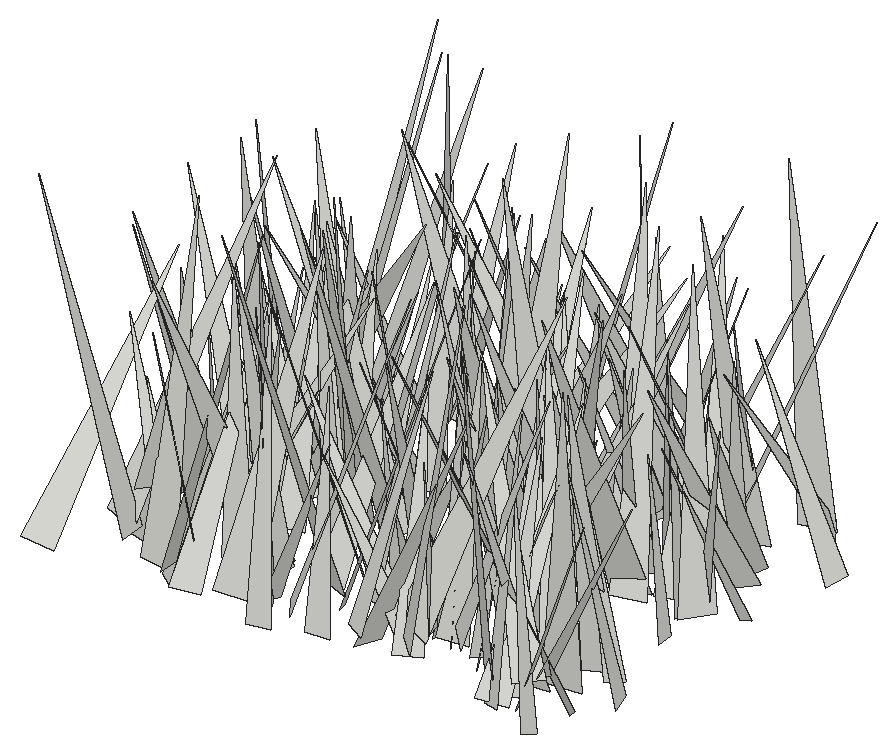
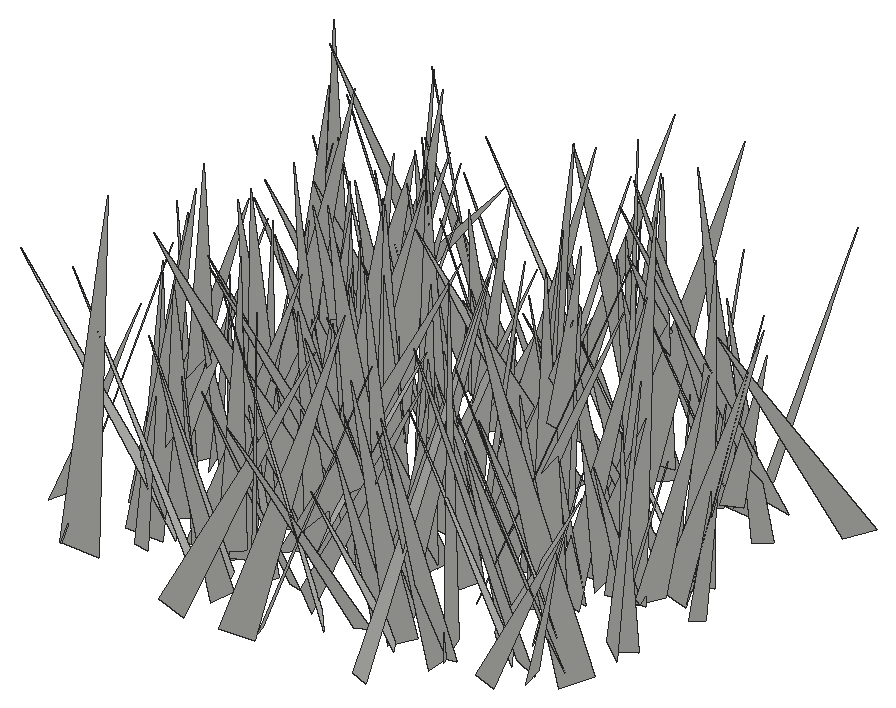
# SketchUp Ruby script. Lengths in inches.
U = 1.inch
M = Sketchup.active_model
def pt(a) = Geom::Point3d.new(a.map { |v| v * U })
def face(e, loops, mat)
  f = e.add_face(loops[0].map { |a| pt(a) })
  loops[1..].each { |l| e.add_face(l.map { |a| pt(a) }).erase! }
  f.material = f.back_material = mat if mat
  f
end
# faces: each face lists its corners as indices into pts; further lists are holes
def faces(e, pts, list, mat = nil) = list.each { |f| face(e, (f[0].is_a?(Array) ? f : [f]).map { |l| l.map { |i| pts[i] } }, mat) }
# xy, xz, yz: faces in a plane at the given z, y or x. An outline is a flat list of corners, or four numbers for a rectangle; further outlines are holes
def ring(l) = l.size == 4 ? [[l[0], l[1]], [l[2], l[1]], [l[2], l[3]], [l[0], l[3]]] : l.each_slice(2).to_a
def flat(e, list, mat, &to3) = list.each { |f| face(e, (f[0].is_a?(Array) ? f : [f]).map { |l| ring(l).map { |u, v| to3.(u, v) } }, mat) }
def xy(e, z, list, mat = nil) = flat(e, list, mat) { |x, y| [x, y, z] }
def xz(e, y, list, mat = nil) = flat(e, list, mat) { |x, z| [x, y, z] }
def yz(e, x, list, mat = nil) = flat(e, list, mat) { |y, z| [x, y, z] }
def lines(e, pts, list) = list.each { |a, b| e.add_line(pt(pts[a]), pt(pts[b])) }
# prism: a flat outline (further loops are holes) pulled along v
def prism(e, loops, v, mat = nil)
  f = face(e, loops, mat); d = Geom::Vector3d.new(v.map { |x| x * U })
  f.pushpull(f.normal.samedirection?(d) ? d.length : -d.length)
end
def box(e, o, s, mat = nil) = prism(e, [[o, [o[0] + s[0], o[1], o[2]], [o[0] + s[0], o[1] + s[1], o[2]], [o[0], o[1] + s[1], o[2]]]], [0, 0, s[2]], mat)
def at(x, y, z, deg = 0) = Geom::Transformation.translation(pt([x, y, z])) * Geom::Transformation.rotation(ORIGIN, Z_AXIS, deg.degrees)
def axes(o, x, y, z) = Geom::Transformation.new([*x, 0, *y, 0, *z, 0, *pt(o).to_a, 1])
def part(name) = M.definitions.add(name)
# library, detail: a bought-in or finely detailed component or shape, given as its bounding box
def library(name, o, s) = part(name).tap { |d| box(d.entities, o, s) }
def detail(e, o, s) = box(e.add_group.entities, o, s)
def put(e, d, t, mat = nil) = e.add_instance(d, t).tap { |i| i.material = mat if mat }
def group(e, t, mat = nil) = e.add_group.tap { |g| g.transformation = t; g.material = mat if mat }.entities
root = M.entities
c1 = part("fur_instance\#9")
p = [[0.8125,0,1.79],[0.67,-0.02,1.48],[0,-0.11,0],[0,0.11,0]]
faces(c1.entities,p,[[0,1,2,3]])
put(root,c1,axes([119.71,154.68,-28.22],[3.07442,-7.15508,0.96712],[-6.88437,-3.22185,-1.95131],[-2.1762,0.08396,7.5392]))
put(root,c1,axes([124.55,151.32,-28.22],[-0.37436,4.96388,1.61425],[5.21969,0.34743,0.14211],[-0.02763,-1.62026,4.97594]))
put(root,c1,axes([133.8,152.13,-28.22],[4.65437,1.55789,0.49043],[1.62302,-4.57734,-0.86283],[-0.1826,-0.97553,4.83174]))
put(root,c1,axes([115.31,151.59,-27.1],[-7.20158,-1.52489,0.67202],[-1.60184,7.15641,-0.92717],[0.45935,1.04894,7.30263]))
put(root,c1,axes([117.04,153.1,-27.1],[-3.29784,-3.61715,1.25797],[-3.53735,3.51322,0.8285],[1.46745,0.33986,4.82422]))
put(root,c1,axes([132.45,151.96,-28.22],[3.92843,5.06138,3.38638],[5.5366,-4.64662,0.52215],[-2.53598,-2.30413,6.38572]))
put(root,c1,axes([119.68,149.32,-27.1],[-3.94963,4.34285,0.40783],[4.0226,3.83915,-1.92507],[1.68683,1.01332,5.54563]))
put(root,c1,axes([124.15,152.97,-27.1],[-4.11377,-6.51171,1.45116],[-6.65439,3.88319,-1.43913],[-0.47668,1.98739,7.56666]))
put(root,c1,axes([122.36,150.46,-28.22],[0.64289,6.12986,1.03372],[6.0316,-0.86662,1.38779],[-1.50455,-0.85491,6.00521]))
put(root,c1,axes([135.55,150.41,-28.22],[-4.92435,-0.05312,0.24709],[-0.15186,4.47527,-2.06445],[0.20202,2.06935,4.47102]))
put(root,c1,axes([121.42,152.375,-28.22],[4.16125,-1.09144,0.28201],[-1.11074,-4.15389,0.31328],[-0.19241,0.37504,4.29058]))
put(root,c1,axes([114.2,153.07,-28.22],[0.76926,-4.66703,1.07076],[-4.59745,-0.41678,1.48633],[1.33832,1.25083,4.49041]))
put(root,c1,axes([127.77,152.92,-28.22],[-4.18794,0.93567,0.33129],[0.9893,4.05153,1.06324],[0.08071,-1.11073,4.15738]))
put(root,c1,axes([126.38,152.1,-28.22],[6.16079,-1.33707,0.34037],[-1.37023,-6.11166,0.79308],[-0.16154,0.84778,6.25413]))
put(root,c1,axes([118.02,150.41,-27.1],[6.46332,2.41268,1.62775],[2.03661,-6.58136,1.66821],[-2.07914,1.05343,6.69422]))
put(root,c1,axes([128.95,151.23,-27.1],[4.76999,5.26227,1.90717],[5.37132,-5.00824,0.38463],[-1.57405,-1.14351,7.09199]))
put(root,c1,axes([126.68,150.94,-27.1],[2.68207,4.86571,0.6841],[4.89534,-2.71316,0.10499],[-0.42283,-0.54794,5.55496]))
put(root,c1,axes([119.82,152.41,-27.1],[-1.05184,5.80364,2.59591],[6.34975,1.09094,0.13387],[0.3189,-2.57972,5.89666]))
put(root,c1,axes([133.72,153.375,-28.22],[-1.08629,-5.09453,1.21583],[-5.17343,0.84989,-1.06105],[-0.81738,1.39139,5.09985]))
put(root,c1,axes([117.41,152.12,-28.22],[-3.05082,2.35934,0.28628],[2.37608,3.01778,0.45074],[-0.05159,-0.53147,3.83025]))
put(root,c1,axes([123.64,150.8,-27.1],[5.3948,4.35682,0.5893],[4.31887,-5.42625,0.57994],[-0.82254,0.08385,6.9101]))
put(root,c1,axes([116.4,151.8,-28.22],[0.76042,7.54721,2.45249],[7.93568,-0.724,-0.23253],[-0.00259,-2.46349,7.58186]))
put(root,c1,axes([121.46,152.47,-28.22],[4.32475,3.25099,2.86901],[3.37923,-5.06616,0.64681],[-2.71679,-1.12634,5.37159]))
put(root,c1,axes([117.27,151.1875,-28.22],[2.99735,3.72962,0.28981],[3.68324,-3.00724,0.60693],[-0.65404,0.15682,4.74613]))
put(root,c1,axes([134.3,153.97,-28.22],[2.16747,-6.96935,1.82134],[-7.20329,-2.08612,0.58967],[0.04123,1.91397,7.27476]))
put(root,c1,axes([128.99,152.79,-27.1],[3.01328,1.01562,1.71575],[1.06477,-3.44849,0.1713],[-1.68569,-0.36275,3.17522]))
put(root,c1,axes([133.1,151.16,-28.22],[2.56304,5.03632,1.18387],[4.82189,-2.80423,1.49027],[-1.87495,-0.32715,5.45094]))
put(root,c1,axes([120.19,151.72,-28.22],[-2.56408,6.91655,2.55207],[6.94878,3.17004,-1.60986],[2.46298,-1.74312,7.19872]))
put(root,c1,axes([130.14,152.91,-27.1],[4.42305,4.26534,0.99754],[4.37397,-4.22348,-1.33498],[0.23791,-1.64944,5.99786]))
put(root,c1,axes([135.9,152.64,-28.22],[-5.38862,-5.55187,0.24968],[-4.68183,4.34761,-4.37054],[-2.99434,3.19341,6.38427]))
put(root,c1,axes([120.52,154.02,-28.22],[-6.63003,0.58928,2.6026],[0.94805,7.03587,0.82207],[2.49439,-1.10786,6.6052]))
put(root,c1,axes([133.06,152.06,-28.22],[-4.05743,3.11883,1.27429],[2.94276,4.25195,-1.03673],[1.64046,0.08657,5.0115]))
put(root,c1,axes([111.75,150.27,-28.22],[-2.9172,5.75801,0.16061],[5.28877,2.74872,-2.48273],[2.2824,0.99014,5.95825]))
put(root,c1,axes([128.23,152.23,-28.22],[-2.91757,4.706,0.99504],[4.75363,2.9987,-0.24403],[0.73452,-0.71423,5.53165]))
put(root,c1,axes([134.27,152.02,-27.1],[-2.5947,5.83184,0.30944],[5.66182,2.42897,1.69778],[-1.43174,-0.96349,6.15308]))
put(root,c1,axes([130.73,153.38,-28.22],[3.30079,2.00098,0.99665],[2.11543,-3.37049,-0.23912],[-0.72261,-0.72685,3.85253]))
put(root,c1,axes([115.67,153.16,-27.1],[-2.80157,3.07223,0.58027],[3.12461,2.72376,0.66487],[-0.11008,-0.87559,4.10431]))
put(root,c1,axes([134.52,152.61,-27.1],[4.0884,0.15219,0.34801],[0.0557,-3.96154,1.07814],[-0.37573,1.0688,3.94662]))
put(root,c1,axes([128.25,152.37,-27.1],[1.6055,7.88479,1.47704],[7.72527,-1.11383,-2.45126],[2.16141,-1.87581,7.66412]))
put(root,c1,axes([123.74,155.37,-28.22],[-4.79453,-5.10071,1.01007],[-5.15614,4.84133,-0.02673],[0.67211,0.75447,7.00029]))
put(root,c1,axes([129.76,155.625,-28.22],[5.66121,2.03663,0.41958],[1.99596,-4.98096,-2.75306],[0.58316,-2.72311,5.34956]))
put(root,c1,axes([136.84,154.43,-28.22],[-4.98874,-1.77944,1.14235],[-1.81158,5.1064,0.04294],[1.09068,0.3424,5.29642]))
put(root,c1,axes([132.96,151.43,-28.22],[-3.49002,4.97532,0.38419],[4.70613,3.43753,-1.76559],[1.65943,0.71499,5.81522]))
put(root,c1,axes([118.51,155.99,-28.22],[-4.19902,-6.23031,2.61813],[-6.01537,4.8505,1.89504],[3.08005,0.97931,7.27031]))
put(root,c1,axes([128.82,154.14,-28.22],[-1.46748,5.77462,2.34569],[6.13429,1.76496,-0.50731],[1.10405,-2.13089,5.93652]))
put(root,c1,axes([128.125,154.48,-28.22],[5.41159,0.09186,1.28906],[0.07062,-5.56242,0.09991],[-1.29039,0.08081,5.41145]))
put(root,c1,axes([134.69,155.86,-28.22],[2.11565,-6.08651,1.80009],[-6.2822,-2.27872,-0.32139],[-0.90548,1.58863,6.43571]))
put(root,c1,axes([117.9,155.93,-28.22],[5.48101,-1.25937,0.85366],[-1.15676,-5.52263,-0.72019],[-0.98826,-0.52035,5.57753]))
put(root,c1,axes([114.3,152.17,-27.1],[2.50136,7.65725,0.1478],[7.63522,-2.48107,-0.67805],[0.59891,-0.35058,8.02686]))
put(root,c1,axes([117.74,154.5,-28.22],[3.45283,2.51437,0.03768],[2.48973,-3.40925,-0.65094],[0.3531,-0.54815,4.22141]))
put(root,c1,axes([124.81,155.34,-28.22],[-4.21656,2.08304,0.19454],[2.06998,4.09043,1.06765],[-0.30342,-1.04195,4.58024]))
put(root,c1,axes([129.93,157.18,-28.22],[-3.59271,-3.52154,0.36411],[-3.38524,3.56898,1.11534],[1.03633,-0.55007,4.90559]))
put(root,c1,axes([135.59,155.59,-28.22],[1.42768,-3.34431,1.65268],[-3.54003,-1.77266,-0.52903],[-1.17641,1.27565,3.59761]))
put(root,c1,axes([125.07,157.35,-28.22],[-0.67207,-6.04885,0.74296],[-6.03248,0.76649,0.78356],[0.86591,0.6451,6.03542]))
put(root,c1,axes([131,156.88,-28.22],[-0.74587,-6.40704,1.23448],[-6.45249,0.53969,-1.09751],[-0.96927,1.33753,6.35625]))
put(root,c1,axes([113.98,157.4,-28.22],[4.76035,-4.27512,0.72339],[-4.20428,-4.81383,-0.78223],[-1.06017,-0.10597,6.35025]))
put(root,c1,axes([128.85,154.05,-28.22],[5.31118,5.11176,2.74997],[4.78098,-5.96627,1.85658],[-3.29161,-0.41778,7.13385]))
put(root,c1,axes([130.91,155.34,-28.22],[-7.32876,-0.97242,0.83606],[-1.07916,7.29688,-0.97277],[0.69283,1.07947,7.32872]))
put(root,c1,axes([123.52,157.71,-28.22],[-2.25691,-7.5793,1.44794],[-7.71352,2.17504,-0.63772],[-0.20948,1.56823,7.88243]))
put(root,c1,axes([126.92,156.79,-28.22],[-3.55918,-3.90599,0.48478],[-3.91702,3.45103,-0.95229],[-0.38568,0.99656,5.19785]))
put(root,c1,axes([130.33,153.8,-28.22],[1.86893,4.92203,0.04113],[4.36091,-1.67616,2.42774],[-2.28266,0.8277,4.67176]))
put(root,c1,axes([126.48,157.73,-28.22],[4.05285,-0.43746,0.41546],[-0.3233,-3.95717,-1.01285],[-0.50937,-0.96903,3.94856]))
put(root,c1,axes([124.16,156.61,-28.22],[0.90627,3.33198,1.59944],[3.57947,-1.20149,0.47479],[-0.9207,-1.39138,3.42023]))
put(root,c1,axes([113.74,158.14,-28.22],[-5.14482,-3.13912,1.24988],[-3.04737,5.29445,0.7535],[1.4594,-0.01101,5.97959]))
put(root,c1,axes([115.6,156.49,-28.22],[-3.72029,-1.54775,1.40082],[-1.82397,3.80239,-0.64288],[1.01535,1.15959,3.97778]))
put(root,c1,axes([132.49,155.91,-28.22],[-2.14866,5.91991,1.32548],[6.06222,2.04254,0.70466],[-0.22751,-1.48381,6.25824]))
put(root,c1,axes([123.9,153.63,-28.22],[6.2923,4.31715,0.79405],[3.75537,-6.01297,2.93303],[-2.27277,2.01685,7.04472]))
put(root,c1,axes([119.83,159.88,-28.22],[-1.88375,-7.99896,1.23534],[-7.80751,2.13018,1.88761],[2.13359,0.73274,7.99805]))
put(root,c1,axes([126.28,157.98,-28.22],[4.01557,-5.25956,2.05629],[-5.53772,-4.16187,0.169],[-1.10676,1.74125,6.61508]))
put(root,c1,axes([124.33,154.78,-28.22],[3.92721,6.27569,0.86047],[6.07775,-4.01843,1.56873],[-1.78486,0.12492,7.23508]))
put(root,c1,axes([127.15,160.48,-28.22],[4.78768,-6.87101,0.53821],[-6.76798,-4.81092,-1.21319],[-1.30189,-0.25808,8.28619]))
put(root,c1,axes([114.15,158.61,-28.22],[-0.64276,-5.9949,1.38637],[-6.03632,0.34404,-1.31091],[-1.1932,1.48889,5.88502]))
put(root,c1,axes([122.42,154.625,-28.22],[-4.56425,4.1816,0.8559],[3.58274,4.43445,-2.55936],[2.31998,1.37862,5.63629]))
put(root,c1,axes([116.25,156.52,-28.22],[2.28513,5.39499,0.34939],[5.12885,-2.04337,-1.99232],[1.70965,-1.08097,5.50984]))
put(root,c1,axes([112.37,159.34,-28.22],[4.01864,-1.00258,0.99057],[-0.63294,-3.95809,-1.43832],[-1.25928,-1.21004,3.88405]))
put(root,c1,axes([121.36,157.57,-28.22],[-6.31517,-2.67121,2.41272],[-3.08957,6.52254,-0.86542],[1.84694,1.77736,6.80204]))
put(root,c1,axes([128.8125,158.05,-28.22],[4.74645,-3.63152,0.20608],[-3.44873,-4.38539,2.15263],[1.15614,1.82746,5.57521]))
put(root,c1,axes([121.21,156.54,-28.22],[-6.71,0.21588,0.88951],[-0.0468,6.49159,-1.92847],[0.91413,1.91692,6.43053]))
put(root,c1,axes([118.56,157.11,-28.22],[-1.85743,4.94831,0.92273],[4.99711,1.93095,-0.29602],[0.60509,-0.75691,5.27714]))
put(root,c1,axes([131.72,161.43,-28.22],[2.00321,-7.73932,0.37509],[-7.71802,-2.02729,-0.61059],[-0.68548,0.20889,7.97102]))
put(root,c1,axes([123.2,159.25,-28.22],[1.52564,-3.34819,0.07276],[-3.07421,-1.36842,1.48995],[1.32851,0.67846,3.36423]))
put(root,c1,axes([129.36,159.05,-28.22],[-2.05605,-4.2865,1.82271],[-4.5186,2.31917,0.35698],[1.13077,1.47345,4.74068]))
put(root,c1,axes([115.48,159.86,-28.22],[1.30407,-7.61557,2.3618],[-7.95747,-1.39423,-0.10194],[-0.50366,2.30972,7.72574]))
put(root,c1,axes([130.09,158.49,-28.22],[2.97809,2.23148,0.68885],[2.24903,-3.04112,0.12836],[-0.62921,-0.30835,3.71915]))
put(root,c1,axes([130.51,156.68,-28.22],[-3.78371,6.02543,0.57396],[5.96039,3.82698,-0.88298],[1.05307,-0.01122,7.05993]))
put(root,c1,axes([122.22,160.31,-28.22],[-3.95359,-4.39819,1.62013],[-4.4402,4.19331,0.54823],[1.50116,0.81969,5.8885]))
put(root,c1,axes([135.09,159.27,-28.22],[-3.75742,-0.36081,1.22113],[-0.40687,3.94545,-0.08619],[1.20657,0.20686,3.77372]))
put(root,c1,axes([128.77,161.64,-28.22],[1.34944,-6.66989,1.0863],[-6.57389,-1.5523,-1.36482],[-1.56569,0.76902,6.66676]))
put(root,c1,axes([128.64,158.72,-28.22],[-2.07994,4.49979,1.08625],[4.57933,2.1742,-0.23818],[0.67657,-0.88257,4.95151]))
put(root,c1,axes([128.86,162,-28.22],[3.45501,-4.88886,0.26504],[-4.85303,-3.46254,-0.60598],[-0.64754,-0.13474,5.95575]))
put(root,c1,axes([114.7,159.34,-28.22],[-5.78073,2.46703,0.60773],[2.49572,5.79658,0.20851],[0.47643,-0.43109,6.28168]))
put(root,c1,axes([122.02,159.32,-28.22],[-1.88222,6.06948,1.49765],[6.0067,1.32242,2.18977],[-1.73238,-2.00921,5.96542]))
put(root,c1,axes([117.15,161.375,-28.22],[-1.29627,-6.42722,1.30707],[-6.54569,1.18361,-0.67151],[-0.41416,1.4099,6.52216]))
put(root,c1,axes([116.67,161.05,-28.22],[3.94876,4.2171,2.00571],[4.64379,-3.26946,-2.26834],[0.4919,-2.98768,5.31331]))
put(root,c1,axes([119.9,163.24,-28.22],[-6.16351,-3.9605,0.27898],[-3.73191,5.95492,2.08903],[1.35509,-1.6142,7.02213]))
put(root,c1,axes([128.67,161.89,-28.22],[3.0521,-3.8403,0.46149],[-3.78154,-3.08617,-0.67208],[-0.8129,-0.06212,4.85917]))
put(root,c1,axes([117.58,159.29,-28.22],[-2.49681,4.68547,0.3153],[4.52882,2.308,1.56527],[-1.24213,-1.0033,5.07323]))
put(root,c1,axes([119.26,160.23,-28.22],[3.71191,-5.65782,4.04126],[-6.28277,-4.69165,-0.79764],[-2.97818,2.84578,6.7196]))
put(root,c1,axes([130.11,159.36,-28.22],[-3.95695,1.67084,0.9926],[1.45221,4.03835,-1.00857],[1.29152,0.5783,4.17516]))
put(root,c1,axes([120.74,160.68,-28.22],[-7.40149,0.22253,0.007],[0.22253,7.40149,0.00759],[0.00677,-0.0078,7.40483]))
put(root,c1,axes([117.37,162.16,-28.22],[5.14782,-4.26055,1.16689],[-4.27581,-5.25589,-0.32723],[-1.10966,0.4872,6.67423]))
put(root,c1,axes([127.77,162.71,-28.22],[7.05622,-1.23215,0.51957],[-1.10047,-6.93599,-1.50315],[-0.75967,-1.39725,7.0035]))
put(root,c1,axes([114.68,161.1875,-28.22],[-3.79015,-1.11399,0.60809],[-1.15598,3.82064,-0.20588],[0.52388,0.37109,3.9451]))
put(root,c1,axes([134.41,162.47,-28.22],[-1.98967,-4.65459,1.69235],[-4.24096,2.54317,2.00863],[2.55803,0.59592,4.64644]))
put(root,c1,axes([125.39,162.07,-28.22],[0.0585,-4.06465,0.78718],[-4.11626,0.02739,0.44734],[0.44434,0.78888,4.04038]))
put(root,c1,axes([130.58,162.91,-28.22],[-0.89521,-5.51634,1.09126],[-5.41102,1.14576,1.35291],[1.53027,0.82431,5.42227]))
put(root,c1,axes([114.91,160.12,-28.22],[-3.70619,1.07071,1.22273],[0.63141,3.75399,-1.37341],[1.4976,1.06701,3.605]))
put(root,c1,axes([127.24,162.42,-28.22],[3.59874,-6.83955,3.08177],[-7.12327,-4.18751,-0.97538],[-2.35281,2.21652,7.66674]))
put(root,c1,axes([125.36,161.66,-28.22],[-2.45983,6.23998,3.07468],[6.83629,2.77173,-0.15592],[1.28687,-2.79677,6.7055]))
put(root,c1,axes([112.89,162.89,-28.22],[0.91273,-4.1627,0.50654],[-4.12867,-0.80133,0.85424],[0.734,0.66898,4.1751]))
put(root,c1,axes([116.97,159.14,-28.22],[-5.60466,1.1961,0.32776],[0.92969,5.05609,-2.5538],[0.82084,2.4404,5.13039]))
put(root,c1,axes([124.52,162.26,-28.22],[7.01983,-0.71592,2.31882],[-0.6287,-7.39114,-0.37866],[-2.34397,-0.1616,7.04608]))
put(root,c1,axes([134.81,164.43,-28.22],[2.61621,-5.42084,0.25429],[-5.22177,-2.59146,-1.52055],[-1.47757,-0.43991,5.82391]))
put(root,c1,axes([136.47,162.45,-28.22],[-1.27388,-3.61865,0.59779],[-3.46584,0.98064,-1.44951],[-1.19998,1.0092,3.55195]))
put(root,c1,axes([124.6875,159.98,-28.22],[-0.78819,5.89997,0.04998],[5.7265,0.75282,1.4401],[-1.42105,-0.23877,5.77555]))
put(root,c1,axes([118.28,161.37,-28.22],[-1.7521,4.37342,1.24469],[4.49457,1.86786,-0.23622],[0.6891,-1.06311,4.7054]))
put(root,c1,axes([134.89,161.49,-28.22],[-6.12251,3.37612,2.03098],[3.42132,6.417,-0.35327],[1.95387,-0.65732,6.98272]))
put(root,c1,axes([123.3,162.42,-28.22],[-0.9402,5.50023,2.63792],[6.09336,0.97222,0.14463],[0.28664,-2.62629,5.57814]))
put(root,c1,axes([122.62,162.35,-28.22],[4.20762,-3.32651,0.12048],[-3.15177,-3.91891,1.86887],[1.07075,1.53645,5.02763]))
put(root,c1,axes([128.79,160.3125,-28.22],[2.4518,5.85296,0.01413],[5.81055,-2.43218,-0.76857],[0.70347,-0.30989,6.29903]))
put(root,c1,axes([131.66,163.125,-28.22],[-0.88602,-4.48963,1.06047],[-4.46813,0.56653,-1.33464],[-1.14769,1.26043,4.37728]))
put(root,c1,axes([117.72,161.5625,-28.22],[4.17653,-0.25853,0.87813],[-0.4857,-4.1025,1.10224],[-0.77592,1.17643,4.03674]))
put(root,c1,axes([134.42,161.11,-28.22],[-5.22043,-0.84385,1.05571],[-1.17009,4.93002,-1.84535],[0.67639,2.01552,4.95577]))
put(root,c1,axes([131.96,160.95,-28.22],[-1.2461,7.24945,1.28302],[7.36015,1.19663,0.38699],[-0.1701,-1.32928,7.34558]))
put(root,c1,axes([128.54,161.49,-28.22],[-3.66348,3.88372,0.60062],[3.90017,3.69385,-0.09601],[0.48235,-0.37054,5.33808]))
put(root,c1,axes([132.22,162.94,-28.22],[4.15283,1.56186,1.94961],[1.7605,-4.5132,-0.13443],[-1.7723,-0.82343,4.43479]))
put(root,c1,axes([134.49,165.39,-28.22],[4.609,-3.3139,0.05026],[-3.15306,-4.41083,-1.68231],[-1.0211,-1.33793,5.42168]))
put(root,c1,axes([133.01,161.88,-28.22],[-1.57636,3.66287,0.67143],[3.67727,1.64614,-0.34684],[0.58749,-0.47537,3.97256]))
put(root,c1,axes([125.1875,163.32,-28.22],[4.4628,-4.8312,0.78242],[-4.8199,-4.15484,1.83716],[0.84924,1.80724,6.31521]))
put(root,c1,axes([126.52,163.34,-28.22],[3.82808,-2.96393,0.87418],[-3.08142,-3.76593,0.72521],[-0.23226,1.11183,4.78677]))
put(root,c1,axes([128.93,163.4375,-28.22],[3.70956,-2.15387,1.10856],[-2.28011,-3.78925,0.26761],[-0.81802,0.79458,4.28116]))
put(root,c1,axes([123.57,163.13,-28.22],[-3.05036,2.77962,1.08054],[2.93347,3.07501,0.37088],[0.53722,-1.00823,4.11016]))
put(root,c1,axes([113.43,163.22,-28.22],[-3.6941,-4.73944,2.34113],[-5.23892,3.66336,-0.85037],[0.70493,2.38895,5.94858]))
put(root,c1,axes([133.71,165.77,-28.22],[-3.10911,-5.59083,0.18925],[-5.58666,3.11434,0.22319],[0.28707,0.05678,6.39328]))
put(root,c1,axes([127.66,164.66,-28.22],[-7.5943,2.08618,0.38061],[2.11361,7.33132,1.9887],[-0.17228,-2.01745,7.62041]))
put(root,c1,axes([116.26,164.46,-28.22],[-3.02688,-2.08558,0.64094],[-2.07151,3.09116,0.27563],[0.68504,0.13224,3.66547]))
put(root,c1,axes([112.98,165.95,-28.22],[2.01455,-7.63294,0.11302],[-6.59973,-1.68273,3.99311],[3.83642,1.11337,6.80994]))
put(root,c1,axes([122.57,165.05,-28.22],[-6.83352,3.26319,2.339],[3.80782,6.73136,1.73366],[1.27275,-2.61852,7.37155]))
put(root,c1,axes([130.33,162.99,-28.22],[-5.59489,5.13542,2.2708],[5.22691,5.9344,-0.54239],[2.05147,-1.11455,7.57503]))
put(root,c1,axes([118.36,162.66,-28.22],[5.33264,0.16428,1.51785],[-0.27785,-5.31816,1.55174],[-1.50122,1.56784,5.10452]))
put(root,c1,axes([120.87,162.73,-28.22],[-5.25856,3.05312,1.43062],[2.8843,5.44607,-1.02073],[1.74617,0.1987,5.99435]))
put(root,c1,axes([126.7,164.37,-28.22],[3.66382,-3.28739,1.57998],[-3.52995,-3.75957,0.36325],[-0.918,1.33625,4.90903]))
put(root,c1,axes([128.91,166.47,-28.22],[4.74802,-2.11154,0.82126],[-1.70244,-4.58339,-1.94189],[-1.49491,-1.48682,4.81989]))
put(root,c1,axes([124.53,162.95,-28.22],[1.506,6.6666,0.93752],[6.04421,-0.91584,-3.19677],[2.9648,-1.51928,6.04088]))
put(root,c1,axes([127.18,164.1,-28.22],[-5.46904,-3.01802,0.13387],[-2.92547,5.22183,-1.79189],[-0.75368,1.63119,5.98398]))
put(root,c1,axes([122.82,164.88,-28.22],[0.6303,-6.24139,2.24897],[-6.57772,-0.29373,1.02832],[0.86396,2.31708,6.18828]))
put(root,c1,axes([124.12,163.9375,-28.22],[-3.47776,6.78239,3.15196],[7.08859,4.09761,-0.99596],[2.38486,-2.28893,7.55669]))
put(root,c1,axes([130.62,166.66,-28.22],[3.32641,-4.64571,1.36805],[-4.19977,-3.59363,-1.99171],[-2.41165,-0.14974,5.35544]))
put(root,c1,axes([118.1,163.82,-28.22],[-0.0874,4.08723,0.80677],[4.1529,0.14964,-0.30818],[0.33125,-0.79758,4.07653]))
put(root,c1,axes([117.39,165.28,-28.22],[-2.7303,-2.91554,0.15676],[-2.8364,2.59761,-1.08937],[-0.69267,0.85529,3.84294]))
put(root,c1,axes([133.33,165.9,-28.22],[0.51611,-4.80053,1.29544],[-4.96034,-0.40702,0.46794],[0.34389,1.33374,4.80546]))
put(root,c1,axes([124.84,163.02,-28.22],[-3.56356,5.20391,0.71647],[5.00613,3.62664,-1.4419],[1.59144,0.24443,6.14008]))
put(root,c1,axes([127.62,162.71,-28.22],[7.47799,-1.52657,1.95795],[-2.25093,-6.79047,3.30259],[-1.04752,3.69369,6.88067]))
put(root,c1,axes([126.9375,166.9,-28.22],[4.19489,0.81761,0.41517],[0.91291,-3.90671,-1.53042],[-0.08632,-1.58339,3.99042]))
put(root,c1,axes([135.03,169.72,-28.22],[-4.76497,-3.93422,0.44703],[-3.2824,4.31602,2.99679],[2.21445,-2.06803,5.40391]))
put(root,c1,axes([129.08,166.8,-28.22],[5.69628,-2.00129,2.37758],[-1.98509,-6.1627,-0.4314],[-2.39112,0.34864,6.02217]))
put(root,c1,axes([132.97,167.25,-28.22],[0.92373,-7.0899,2.33425],[-7.39568,-1.18748,-0.68009],[-1.00963,2.21177,7.11741]))
put(root,c1,axes([132.43,168.1,-28.22],[-2.364,-4.99525,1.36106],[-4.8414,2.66304,1.36474],[1.83462,0.59091,5.35523]))
put(root,c1,axes([137.35,166.92,-28.22],[-5.10669,0.68056,0.36828],[0.71376,5.09217,0.48729],[0.29888,-0.53268,5.12875]))
put(root,c1,axes([120.9,166.01,-28.22],[4.30125,1.72732,0.68489],[1.69718,-4.35514,0.32517],[-0.75649,0.05042,4.6237]))
put(root,c1,axes([132.66,165.44,-28.22],[-4.49131,4.50007,0.95246],[4.50728,4.57122,-0.34355],[0.91773,-0.42777,6.34858]))
put(root,c1,axes([114.98,164.26,-28.22],[5.00071,5.94343,0.88428],[5.7504,-5.06729,1.53914],[-1.74336,0.3341,7.61331]))
put(root,c1,axes([124.92,167.4375,-28.22],[-3.40667,-4.88664,0.79026],[-4.79108,3.01371,-2.01797],[-1.2447,1.77411,5.60468]))
put(root,c1,axes([118.2,167.02,-28.22],[7.01213,2.59998,3.36264],[2.81322,-7.70163,0.08845],[-3.18638,-1.07803,7.47811]))
put(root,c1,axes([119.61,170.87,-28.22],[-4.53794,-6.8341,0.16977],[-6.57814,4.42074,2.12406],[1.86058,-1.03861,7.92377]))
put(root,c1,axes([130.82,166.66,-28.22],[-3.597,-0.64897,1.74683],[-0.97146,3.89365,-0.55385],[1.59023,0.91068,3.61287]))
put(root,c1,axes([120.08,167.62,-28.22],[4.08731,-3.32744,0.79787],[-3.41978,-4.01464,0.77613],[-0.11643,1.10699,5.21302]))
put(root,c1,axes([116.09,165.96,-28.22],[4.71146,3.59222,0.48874],[3.58656,-4.73541,0.23065],[-0.52868,-0.11206,5.92019]))
put(root,c1,axes([121.5,167.03,-28.22],[-0.91828,3.53646,1.4047],[3.57282,1.29857,-0.93362],[1.30946,-1.06309,3.53244]))
put(root,c1,axes([114.51,166.71,-28.22],[-3.94683,-0.00707,0.27926],[-0.08275,3.80753,-1.07302],[0.26682,1.07619,3.79817]))
put(root,c1,axes([125.96,166.86,-28.22],[2.1149,3.97719,0.39309],[3.90996,-1.96694,-1.13523],[0.82754,-0.87089,4.35914]))
put(root,c1,axes([115.73,168.08,-28.22],[-0.24742,-3.68689,1.2628],[-3.55064,-0.30834,-1.59591],[-1.60648,1.24932,3.33279]))
put(root,c1,axes([115.16,166.28,-28.22],[3.5873,6.66463,1.07182],[6.75002,-3.55215,-0.50434],[-0.05834,-1.18311,7.55193]))
put(root,c1,axes([124.87,170.33,-28.22],[-4.86193,-2.9811,0.43497],[-2.74592,4.72474,1.68858],[1.2394,-1.22654,5.44739]))
put(root,c1,axes([128.29,167.84,-28.22],[4.75078,2.28793,0.55209],[2.32197,-4.75936,-0.25743],[-0.38451,-0.47246,5.26671]))
put(root,c1,axes([117.97,168.15,-28.22],[4.91416,0.05831,0.74386],[0.02898,-4.96646,0.19783],[-0.74558,0.19125,4.91052]))
put(root,c1,axes([125.35,171.14,-28.22],[3.27903,-5.74844,0.73311],[-5.41958,-3.34021,-1.9507],[-2.05188,-0.36394,6.32387]))
put(root,c1,axes([132.375,166.05,-28.22],[5.97415,4.42308,0.10738],[4.35531,-5.91092,1.16532],[-0.77872,0.87356,7.3414]))
put(root,c1,axes([114.27,165.34,-28.22],[3.79972,6.90357,0.39781],[6.61789,-3.76205,2.07507],[-2.00527,0.66563,7.60206]))
put(root,c1,axes([128.59,171.08,-28.22],[0.00181,-5.98408,0.19016],[-5.68264,-0.06159,-1.88392],[-1.88493,0.17992,5.67979]))
put(root,c1,axes([118.11,167.63,-28.22],[-0.03084,5.75903,1.17934],[5.85206,0.14189,-0.53988],[0.55736,-1.17118,5.73375]))
put(root,c1,axes([128.97,168.89,-28.22],[5.75926,3.61485,0.22209],[3.58079,-5.62103,-1.36658],[0.54262,-1.27375,6.66098]))
put(root,c1,axes([126.74,168.42,-28.22],[-5.7993,-3.05465,2.69516],[-3.68736,5.92923,-1.21419],[1.7315,2.39584,6.44116]))
put(root,c1,axes([121.92,167.76,-28.22],[1.05381,5.0713,0.10966],[4.76326,-0.95083,-1.80217],[1.74396,-0.4674,4.856]))
put(root,c1,axes([120.24,167.9,-28.22],[3.43862,2.40363,0.16823],[2.31203,-3.37399,0.94893],[-0.67841,0.6845,4.08669]))
put(root,c1,axes([123.48,168.26,-28.22],[5.53821,4.98185,1.27941],[5.04776,-5.62536,0.05401],[-0.98782,-0.81487,7.449]))
put(root,c1,axes([127.62,169.21,-28.22],[4.66394,-1.20705,1.00362],[-1.36601,-4.67089,0.73033],[-0.77347,0.97077,4.76192]))
put(root,c1,axes([134.16,169.71,-28.22],[0.36283,-7.33481,3.26148],[-7.98321,-0.67122,-0.62142],[-0.83968,3.21222,7.31744]))
